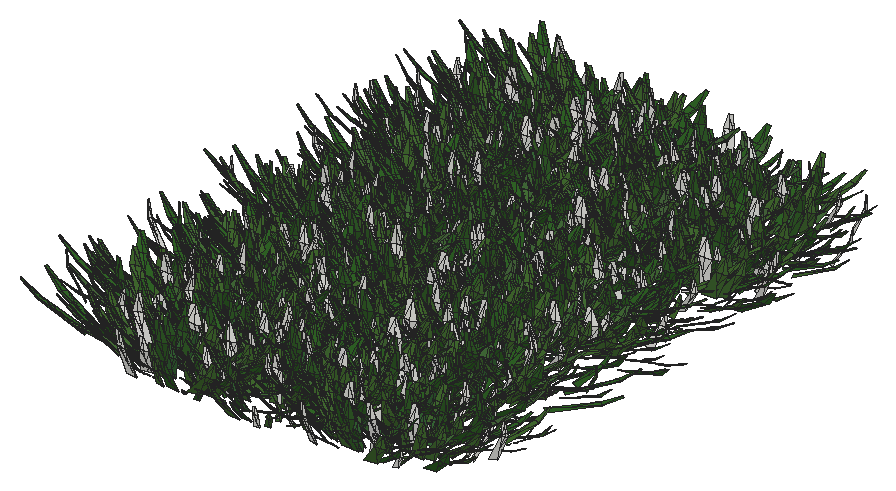
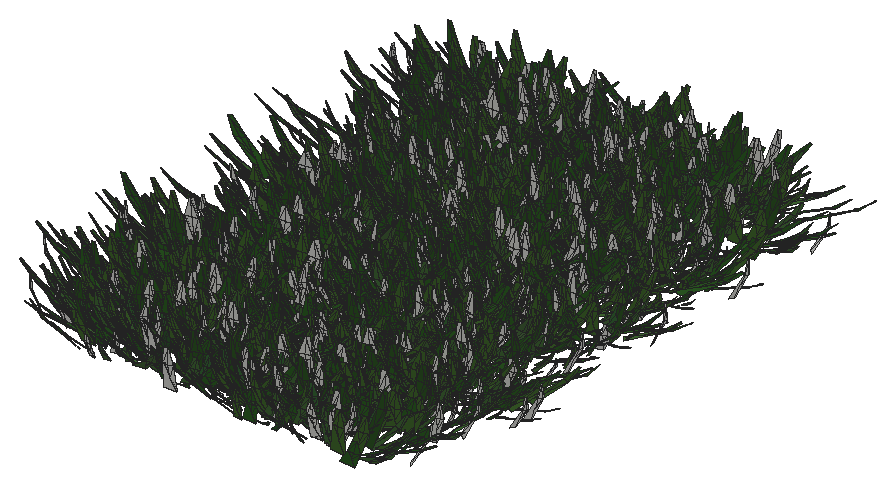
# SketchUp Ruby script. Lengths in inches.
U = 1.inch
M = Sketchup.active_model
def pt(a) = Geom::Point3d.new(a.map { |v| v * U })
def face(e, loops, mat)
  f = e.add_face(loops[0].map { |a| pt(a) })
  loops[1..].each { |l| e.add_face(l.map { |a| pt(a) }).erase! }
  f.material = f.back_material = mat if mat
  f
end
# faces: each face lists its corners as indices into pts; further lists are holes
def faces(e, pts, list, mat = nil) = list.each { |f| face(e, (f[0].is_a?(Array) ? f : [f]).map { |l| l.map { |i| pts[i] } }, mat) }
# xy, xz, yz: faces in a plane at the given z, y or x. An outline is a flat list of corners, or four numbers for a rectangle; further outlines are holes
def ring(l) = l.size == 4 ? [[l[0], l[1]], [l[2], l[1]], [l[2], l[3]], [l[0], l[3]]] : l.each_slice(2).to_a
def flat(e, list, mat, &to3) = list.each { |f| face(e, (f[0].is_a?(Array) ? f : [f]).map { |l| ring(l).map { |u, v| to3.(u, v) } }, mat) }
def xy(e, z, list, mat = nil) = flat(e, list, mat) { |x, y| [x, y, z] }
def xz(e, y, list, mat = nil) = flat(e, list, mat) { |x, z| [x, y, z] }
def yz(e, x, list, mat = nil) = flat(e, list, mat) { |y, z| [x, y, z] }
def lines(e, pts, list) = list.each { |a, b| e.add_line(pt(pts[a]), pt(pts[b])) }
# prism: a flat outline (further loops are holes) pulled along v
def prism(e, loops, v, mat = nil)
  f = face(e, loops, mat); d = Geom::Vector3d.new(v.map { |x| x * U })
  f.pushpull(f.normal.samedirection?(d) ? d.length : -d.length)
end
def box(e, o, s, mat = nil) = prism(e, [[o, [o[0] + s[0], o[1], o[2]], [o[0] + s[0], o[1] + s[1], o[2]], [o[0], o[1] + s[1], o[2]]]], [0, 0, s[2]], mat)
def at(x, y, z, deg = 0) = Geom::Transformation.translation(pt([x, y, z])) * Geom::Transformation.rotation(ORIGIN, Z_AXIS, deg.degrees)
def axes(o, x, y, z) = Geom::Transformation.new([*x, 0, *y, 0, *z, 0, *pt(o).to_a, 1])
def part(name) = M.definitions.add(name)
# library, detail: a bought-in or finely detailed component or shape, given as its bounding box
def library(name, o, s) = part(name).tap { |d| box(d.entities, o, s) }
def detail(e, o, s) = box(e.add_group.entities, o, s)
def put(e, d, t, mat = nil) = e.add_instance(d, t).tap { |i| i.material = mat if mat }
def group(e, t, mat = nil) = e.add_group.tap { |g| g.transformation = t; g.material = mat if mat }.entities
root = M.entities
M.materials.add("Material82").color = [68, 110, 58]
M.materials.add("Material83").color = [48, 90, 38]
M.materials.add("Material84").color = [68, 110, 48]
M.materials.add("Material85").color = [48, 90, 48]
M.materials.add("Material86").color = [58, 110, 58]
M.materials.add("Material87").color = [58, 90, 38]
M.materials.add("Material88").color = [68, 100, 58]
M.materials.add("Material89").color = [48, 100, 38]
c1 = part("grass00")
p = [[-0.6875,0.15,0],[-0.56,0.08,5.52],[-0.04,0.03,2.76],[0.48,-0.02,0],[0.35,-0.02,5.52],[-0.1,-0.14,5.52],
  [-0.12,0.65,8.37],[-0.42,0.65,8.37]]
faces(c1.entities,p,[[0,1,2,3],[3,2,4],[1,5,2],[5,4,2],[1,6,5],[4,5,6],[7,6,1]])
c2 = part("Group16\#1")
put(c2.entities,c1,axes([1.44,-0.61,-0.01],[0.05352,0.12609,0],[-0.10704,0.04543,0.07239],[0.06664,-0.02828,0.11628]),"Material85")
put(c2.entities,c1,axes([0.76,-0.15,-0.01],[0.04676,0.24062,0],[-0.23162,0.04501,0.06642],[0.0652,-0.01267,0.23595]),"Material82")
put(c2.entities,c1,axes([0.79,0.01,-0.01],[-0.00606,0.34651,0],[-0.34381,-0.00602,0.0432],[0.04319,0.00076,0.34386]))
put(c2.entities,c1,axes([1,0.23,-0.01],[-0.07192,0.31144,0],[-0.28722,-0.06632,0.1236],[0.12043,0.02781,0.29478]),"Material84")
put(c2.entities,c1,axes([1.66,0.77,-0.01],[-0.13828,0.29651,0],[-0.21551,-0.1005,0.22471],[0.20365,0.09498,0.23779]),"Material89")
put(c2.entities,c1,axes([0.6875,0.52,-0.01],[-0.18126,0.24051,0],[-0.22746,-0.17142,0.09788],[0.07817,0.05891,0.28481]),"Material84")
put(c2.entities,c1,axes([0.68,0.78,-0.01],[-0.215,0.18688,0],[-0.12385,-0.14248,0.21334],[0.13995,0.16101,0.18878]),"Material82")
put(c2.entities,c1,axes([0.56,1,-0.01],[-0.13756,0.07624,0],[-0.06159,-0.11112,0.0927],[0.04494,0.08108,0.12705]),"Material84")
put(c2.entities,c1,axes([0.2,0.64,-0.01],[-0.23729,0.07254,0],[-0.05711,-0.18681,0.153],[0.04473,0.14632,0.19535]),"Material89")
put(c2.entities,c1,axes([0.0625,0.72,-0.01],[-0.28874,0.02525,0],[-0.02179,-0.24916,0.14647],[0.01276,0.14591,0.25012]),"Material82")
put(c2.entities,c1,axes([-0.08,0.62,-0.01],[-0.34089,-0.04187,0],[0.03255,-0.26504,0.216],[-0.02633,0.21439,0.26703]),"Material89")
put(c2.entities,c1,axes([-0.34,0.98,-0.01],[-0.14314,-0.0493,0],[0.04397,-0.12769,0.06843],[-0.02228,0.0647,0.13505]),"Material89")
put(c2.entities,c1,axes([-0.87,1.45,-0.01],[-0.23488,-0.14114,0],[0.13761,-0.22901,0.06087],[-0.03135,0.05217,0.26717]))
put(c2.entities,c1,axes([-0.72,0.77,-0.01],[-0.14208,-0.13251,0],[0.07209,-0.0773,0.16301],[-0.11118,0.11922,0.1057]),"Material89")
put(c2.entities,c1,axes([-0.62,0.43,-0.01],[-0.14845,-0.21203,0],[0.18654,-0.13061,0.12304],[-0.10079,0.07057,0.22772]),"Material82")
put(c2.entities,c1,axes([-0.68,0.29,-0.01],[-0.13639,-0.32136,0],[0.31723,-0.13464,0.05579],[-0.05136,0.0218,0.34462]),"Material83")
put(c2.entities,c1,axes([-0.64,0.125,-0.01],[-0.0458,-0.23569,0],[0.22124,-0.043,0.08276],[-0.08124,0.01579,0.22538]),"Material86")
put(c2.entities,c1,axes([-1.6,-0.03,-0.01],[0.00576,-0.32897,0],[0.27526,0.00482,0.18018],[-0.18015,-0.00315,0.2753]),"Material84")
put(c2.entities,c1,axes([-1.36,-0.31,-0.01],[0.05718,-0.24765,0],[0.18172,0.04196,0.17267],[-0.16825,-0.03885,0.1865]),"Material89")
put(c2.entities,c1,axes([-1.54,-0.72,-0.01],[0.06537,-0.14017,0],[0.13555,0.06321,0.03939],[-0.0357,-0.01665,0.14956]))
put(c2.entities,c1,axes([-1.19,-0.9,-0.01],[0.09597,-0.12735,0],[0.11214,0.08451,0.07557],[-0.06035,-0.04548,0.14042]),"Material88")
put(c2.entities,c1,axes([-0.47,-0.54,-0.01],[0.11588,-0.10072,0],[0.0618,0.0711,0.12124],[-0.07953,-0.0915,0.0942]))
put(c2.entities,c1,axes([-0.47,-0.84,-0.01],[0.11927,-0.0661,0],[0.06603,0.11913,0.00646],[-0.00313,-0.00565,0.13621]),"Material84")
put(c2.entities,c1,axes([-0.38,-1.24,-0.01],[0.28037,-0.08571,0],[0.0618,0.20215,0.20315],[-0.05939,-0.19428,0.21139]),"Material88")
put(c2.entities,c1,axes([-0.06,-0.66,-0.01],[0.22719,-0.01987,0],[0.01247,0.14255,0.17758],[-0.01547,-0.17691,0.1431]),"Material87")
put(c2.entities,c1,axes([0.11,-0.89,-0.01],[0.14882,0.01828,0],[-0.01058,0.08611,0.12229],[0.01491,-0.12138,0.08676]),"Material85")
put(c2.entities,c1,axes([0.25,-0.72,-0.01],[0.20481,0.07053,0],[-0.06206,0.18022,0.10291],[0.03351,-0.0973,0.1906]),"Material85")
put(c2.entities,c1,axes([0.85,-1.42,-0.01],[0.16481,0.09904,0],[-0.09472,0.15762,0.05616],[0.02893,-0.04814,0.18389]),"Material84")
put(c2.entities,c1,axes([1.01,-1.09,-0.01],[0.21858,0.20385,0],[-0.17495,0.1876,0.15339],[0.10462,-0.11218,0.25652]),"Material89")
put(c2.entities,c1,axes([1.01,-0.71,-0.01],[0.08733,0.12473,0],[-0.06445,0.04512,0.13037],[0.1068,-0.07477,0.07867]),"Material85")
c3 = part("Group15\#1")
put(c3.entities,c2,at(0,0,0))
c4 = part("3darcstudiotree_grass00\#1")
put(c4.entities,c3,at(0,0,0))
put(root,c4,axes([746.18,955.9,-29.74],[2.02269,1.40625,0],[-2.88305,0.64496,-0.03898],[-0.27125,0.06068,1.98748]))
put(root,c4,axes([746.54,983.84,-29.74],[2.29641,1.07421,0],[-2.57105,0.85483,-0.04117],[-0.19383,0.06444,1.55213]))
put(root,c4,axes([746.51,946.6,-29.74],[0.20899,1.64265,0],[-4.27343,0.08456,-0.03261],[-0.1888,0.00374,1.85888]))
put(root,c4,axes([746.37,966.71,-29.74],[1.08869,1.44245,0],[-3.40274,0.39943,-0.00785],[-0.05372,0.00631,1.89978]))
put(root,c4,axes([746.58,981.94,-29.74],[2.7006,1.1614,0],[-2.43909,0.8821,-0.03804],[-0.19893,0.07194,1.7602]))
put(root,c4,axes([749.25,973.19,-29.74],[-2.45174,-1.03973,0],[2.50397,-0.91832,-0.03633],[0.18002,-0.06602,1.73438]))
put(root,c4,axes([749.35,970.78,-29.74],[-1.7758,-1.16797,0],[3.11451,-0.73649,-0.04451],[0.21848,-0.05166,1.55797]))
put(root,c4,axes([749.84,960.11,-29.74],[-4.0045,-0.70324,0],[1.53901,-1.36302,-0.04343],[0.08424,-0.0746,1.35201]))
put(root,c4,axes([749.58,953.62,-29.74],[-0.8562,-1.46222,0],[3.2715,-0.29793,-0.0292],[0.1741,-0.01586,1.53984]))
put(root,c4,axes([749.32,961.45,-29.74],[2.12424,-1.58648,0],[2.98317,0.62124,-0.03491],[0.20173,0.04201,1.65255]))
put(root,c4,axes([750.05,942.04,-29.74],[-3.45178,0.2701,0],[-0.90786,-1.80446,-0.05548],[-0.0508,-0.10098,1.6451]))
put(root,c4,axes([751.18,982.04,-29.74],[-3.12186,-1.16816,0],[2.84193,-1.18123,-0.00166],[0.00643,-0.00267,1.74215]))
put(root,c4,axes([749.34,988.83,-29.74],[3.25093,0.54248,0],[-1.41803,1.32165,-0.02719],[-0.07494,0.06985,1.929]))
put(root,c4,axes([749.35,989.51,-29.74],[-0.25702,1.50589,0],[-4.4334,-0.11768,-0.01753],[-0.09867,-0.00262,1.87889]))
put(root,c4,axes([749.26,967.875,-29.74],[3.97101,0.68213,0],[-1.55734,1.41002,-0.04191],[-0.07595,0.06876,1.32656]))
put(root,c4,axes([749.84,995.21,-29.74],[0.4621,1.41992,0],[-4.03416,0.20419,-0.0516],[-0.33532,0.01697,1.99718]))
put(root,c4,axes([749.66,977.52,-29.74],[4.12561,0.29265,0],[-0.72369,1.58676,-0.03729],[-0.0346,0.07587,1.60628]))
put(root,c4,axes([751.41,950.6,-29.74],[-3.96689,-0.26306,0],[0.64548,-1.51387,-0.0114],[0.01279,-0.03,1.97478]))
put(root,c4,axes([749.91,974.62,-29.74],[2.01819,1.66422,0],[-3.45385,0.65143,-0.02212],[-0.1358,0.02561,1.95299]))
put(root,c4,axes([750.19,958.22,-29.74],[-0.26486,1.49696,0],[-3.89065,-0.10706,-0.02357],[-0.1242,-0.00342,1.54387]))
put(root,c4,axes([750.2,948.51,-29.74],[4.24203,-0.02956,0],[0.08072,1.80172,-0.02875],[0.00231,0.05162,1.55972]))
put(root,c4,axes([750.35,983.97,-29.74],[2.46344,0.86677,0],[-2.31784,1.02455,-0.00625],[-0.02756,0.01218,1.72796]))
put(root,c4,axes([751.8,965.53,-29.74],[-3.7951,0.9119,0],[-2.12877,-1.37789,-0.05764],[-0.17628,-0.1141,1.8024]))
put(root,c4,axes([752.19,944.45,-29.74],[1.13972,-1.41461,0],[4.50389,0.56436,-0.03698],[0.18209,0.02282,1.82987]))
put(root,c4,axes([752.75,954.77,-29.74],[-2.49551,-1.26471,0],[2.8619,-0.87828,-0.01663],[0.09126,-0.02801,1.89037]))
put(root,c4,axes([752.39,940.35,-29.74],[-2.98133,1.10226,0],[-2.6348,-1.10837,-0.04557],[-0.21161,-0.08902,1.96028]))
put(root,c4,axes([752,978.84,-29.74],[-2.13819,1.22316,0],[-3.167,-0.86103,-0.02321],[-0.1127,-0.03064,1.70026]))
put(root,c4,axes([752.66,947.39,-29.74],[-3.3677,0.38425,0],[-1.22656,-1.67195,-0.00573],[-0.0077,-0.0105,1.59925]))
put(root,c4,axes([752.61,986.4,-29.74],[2.12809,-1.0558,0],[3.61722,1.13396,-0.06111],[0.24603,0.07713,1.78135]))
put(root,c4,axes([752.72,993.1,-29.74],[3.47556,-0.63984,0],[1.81232,1.53108,-0.02938],[0.06383,0.05392,1.64954]))
put(root,c4,axes([752.54,964.29,-29.74],[4.6709,-0.11713,0],[0.23839,1.47848,-0.03177],[0.01367,0.08477,1.90853]))
put(root,c4,axes([754.75,971.1,-29.74],[-3.65792,-0.8597,0],[1.995,-1.32021,-0.01663],[0.05672,-0.03754,1.94585]))
put(root,c4,axes([754.9,940.4,-29.74],[3.22982,-1.36398,0],[2.52221,0.92889,-0.01281],[0.05669,0.02088,1.56626]))
put(root,c4,axes([756.37,966.21,-29.74],[-1.61628,-1.19973,0],[3.67441,-0.7699,-0.00698],[0.03732,-0.00782,1.8873]))
put(root,c4,axes([756.01,944.1875,-29.74],[1.53079,-1.5017,0],[4.19952,0.6658,-0.01772],[0.08663,0.01374,1.7874]))
put(root,c4,axes([756.53,953.47,-29.74],[-3.12873,-1.31633,0],[2.88309,-1.0658,-0.03051],[0.12402,-0.04585,1.65027]))
put(root,c4,axes([755.92,991.84,-29.74],[2.10607,-1.53284,0],[3.55653,0.76,-0.00988],[0.05409,0.01156,1.88737]))
put(root,c4,axes([754.89,959.43,-29.74],[4.72899,0.01401,0],[-0.03317,1.74196,-0.012],[-0.00046,0.02441,1.70791]))
put(root,c4,axes([755.64,942.24,-29.74],[3.14565,-0.76847,0],[1.85222,1.17921,-0.00486],[0.01386,0.00882,1.42853]))
put(root,c4,axes([755.02,961.83,-29.74],[1.47307,1.52241,0],[-3.55442,0.5349,-0.03212],[-0.18221,0.02742,1.73128]))
put(root,c4,axes([755.39,948.7,-29.74],[3.86384,0.07818,0],[-0.23972,1.84255,-0.05168],[-0.01275,0.09801,1.68853]))
put(root,c4,axes([755.23,955.48,-29.74],[0.17144,1.84869,0],[-4.60552,0.06643,-0.0182],[-0.07619,0.0011,1.44668]))
put(root,c4,axes([755.38,974.37,-29.74],[0.6087,1.43701,0],[-3.38203,0.22281,-0.00028],[-0.00164,0.00011,1.50491]))
put(root,c4,axes([755.7,990.32,-29.74],[-0.11554,1.45354,0],[-4.02615,-0.04978,-0.04067],[-0.20655,-0.00255,1.53414]))
put(root,c4,axes([756.52,981.89,-29.74],[-3.14808,1.22755,0],[-2.57668,-1.02773,-0.03762],[-0.14164,-0.05649,1.47105]))
put(root,c4,axes([755.37,986.65,-29.74],[0.48824,1.58889,0],[-4.56618,0.21822,-0.01569],[-0.06712,0.00321,1.48562]))
put(root,c4,axes([757.53,977.55,-29.74],[-3.3453,-1.30601,0],[3.28392,-1.30825,-0.03717],[0.14464,-0.05762,1.93537]))
put(root,c4,axes([757.32,972.4,-29.74],[-4.03093,-0.26709,0],[0.61626,-1.44652,-0.01654],[0.01865,-0.04378,1.89711]))
put(root,c4,axes([757.72,978.98,-29.74],[-1.63649,-1.29377,0],[3.38922,-0.66676,-0.00448],[0.02699,-0.00531,1.90991]))
put(root,c4,axes([756.9,958.33,-29.74],[-3.19374,0.7238,0],[-2.32014,-1.59223,-0.04948],[-0.1132,-0.07768,1.60238]))
put(root,c4,axes([756.35,984.03,-29.74],[0.67214,1.30105,0],[-3.68417,0.29602,-0.04728],[-0.27019,0.02171,1.64346]))
put(root,c4,axes([756.68,968.28,-29.74],[3.23921,0.6316,0],[-1.61427,1.28761,-0.03066],[-0.08714,0.06951,1.75054]))
put(root,c4,axes([757.78,947.34,-29.74],[0.38628,-1.42854,0],[3.50239,0.14729,-0.04937],[0.32013,0.01346,1.72169]))
put(root,c4,axes([758.01,963.77,-29.74],[-1.61807,1.52118,0],[-3.6405,-0.60227,-0.04701],[-0.26943,-0.04457,1.83905]))
put(root,c4,axes([758.2,951.08,-29.74],[0.41177,1.61489,0],[-3.5087,0.13914,-0.04963],[-0.27633,0.01096,1.47912]))
put(root,c4,axes([757.57,994.14,-29.74],[3.03872,1.12896,0],[-3.11924,1.30579,-0.01047],[-0.04051,0.01696,1.92288]))
put(root,c4,axes([758.61,987.59,-29.74],[3.86781,0.52244,0],[-1.13731,1.30954,-0.02009],[-0.0432,0.04974,1.7458]))
put(root,c4,axes([760.32,986.48,-29.74],[-4.0386,-0.4374,0],[0.94795,-1.36128,-0.02848],[0.0516,-0.0741,1.83531]))
put(root,c4,axes([760.06,992.54,-29.74],[-0.39879,-1.78911,0],[3.98788,-0.13825,-0.04765],[0.27848,-0.00965,1.76037]))
put(root,c4,axes([760.28,995.03,-29.74],[-3.75498,0.92244,0],[-1.75834,-1.11323,-0.01072],[-0.04199,-0.02659,1.84718]))
put(root,c4,axes([760.82,955.28,-29.74],[-3.9685,0.8355,0],[-2.02289,-1.49439,-0.03463],[-0.09424,-0.06962,1.86049]))
put(root,c4,axes([760.41,962.1875,-29.74],[-1.70053,1.52985,0],[-3.13018,-0.54115,-0.01229],[-0.08699,-0.01504,1.9803]))
put(root,c4,axes([761.82,983.63,-29.74],[-3.28059,-1.08182,0],[2.91353,-1.37413,-0.04137],[0.10673,-0.05034,1.36909]))
put(root,c4,axes([761.33,975.17,-29.74],[3.17929,-0.7211,0],[2.23361,1.53163,-0.03788],[0.07878,0.05402,1.40078]))
put(root,c4,axes([760.76,972.49,-29.74],[4.05026,0.33604,0],[-0.7921,1.48485,-0.04482],[-0.0484,0.09073,1.51278]))
put(root,c4,axes([762.53,987.75,-29.74],[-2.84597,-0.98358,0],[2.28129,-1.02662,-0.01406],[0.06335,-0.02851,1.77353]))
put(root,c4,axes([761.69,981.77,-29.74],[3.81863,-0.53813,0],[1.40932,1.55539,-0.0155],[0.0332,0.03664,1.9985]))
put(root,c4,axes([763.01,949.61,-29.74],[-2.42754,-1.16571,0],[2.71881,-0.88058,-0.021],[0.08634,-0.02796,1.40308]))
put(root,c4,axes([762.95,956.96,-29.74],[-1.73285,-1.40976,0],[3.20349,-0.61242,-0.03263],[0.20579,-0.03934,1.87]))
put(root,c4,axes([761.86,979.68,-29.74],[3.58142,-0.447,0],[1.06233,1.32378,-0.04021],[0.07095,0.08841,1.5432]))
put(root,c4,axes([763.12,953.95,-29.74],[-4.30499,0.20084,0],[-0.50439,-1.68151,-0.02284],[-0.01208,-0.04026,1.44864]))
put(root,c4,axes([762.57,946.27,-29.74],[-2.18902,1.07825,0],[-2.9207,-0.92221,-0.02462],[-0.13408,-0.04234,1.95656]))
put(root,c4,axes([762,942.99,-29.74],[2.94971,1.39882,0],[-3.26889,1.07209,-0.02991],[-0.14108,0.04627,1.95467]))
put(root,c4,axes([763.86,964.38,-29.74],[0.02605,-1.38879,0],[4.64619,0.01356,-0.04606],[0.23946,0.0007,1.81052]))
put(root,c4,axes([762.28,966.1,-29.74],[3.34775,0.73741,0],[-1.81639,1.28251,-0.02091],[-0.0568,0.0401,1.55496]))
put(root,c4,axes([762.1875,977.25,-29.74],[4.2068,0.84458,0],[-2.08885,1.6182,-0.01612],[-0.03432,0.02659,1.61949]))
put(root,c4,axes([763.64,969.12,-29.74],[-3.54698,0.73807,0],[-1.81276,-1.35492,-0.01893],[-0.04162,-0.0311,1.37131]))
put(root,c4,axes([763.66,944.96,-29.74],[-3.36311,0.85521,0],[-1.93534,-1.1837,-0.01497],[-0.0443,-0.0271,1.4615]))
put(root,c4,axes([763.03,940.16,-29.74],[0.45304,1.69594,0],[-3.37186,0.14009,-0.01763],[-0.11097,0.00461,1.60818]))
put(root,c4,axes([763.26,970.46,-29.74],[2.84839,1.04367,0],[-2.27167,0.96426,-0.03885],[-0.20657,0.08768,1.95422]))
put(root,c4,axes([763.78,989.98,-29.74],[3.6343,-0.40762,0],[1.19135,1.65202,-0.03545],[0.05267,0.07304,1.77295]))
put(root,c4,axes([763.49,959.63,-29.74],[0.87217,1.79185,0],[-4.36686,0.33058,-0.02457],[-0.1156,0.00875,1.59681]))
put(root,c4,axes([764.07,950.48,-29.74],[3.8213,1.10557,0],[-2.37941,1.27911,-0.00415],[-0.01079,0.0058,1.32509]))
put(root,c4,axes([765.6,955.88,-29.74],[1.36885,-1.43158,0],[3.98655,0.59286,-0.04892],[0.27754,0.04127,1.93615]))
put(root,c4,axes([766.26,975.04,-29.74],[-3.05635,-0.6343,0],[1.70161,-1.2752,-0.01604],[0.05188,-0.03888,1.9024]))
put(root,c4,axes([766.42,983.79,-29.74],[-0.79946,-1.53657,0],[4.27905,-0.34626,-0.03341],[0.18605,-0.01506,1.86102]))
put(root,c4,axes([766.06,953.25,-29.74],[1.53865,-1.45346,0],[4.25105,0.69992,-0.03949],[0.18935,0.03118,1.7941]))
put(root,c4,axes([766.71,967.02,-29.74],[-2.53143,-1.15701,0],[3.22557,-1.09761,-0.03179],[0.10043,-0.03417,1.33245]))
put(root,c4,axes([767.22,978.59,-29.74],[0.41929,-1.46273,0],[4.6699,0.2082,-0.01256],[0.06761,0.00301,1.90836]))
put(root,c4,axes([765.6875,945.1,-29.74],[3.57437,0.42668,0],[-1.04232,1.35805,-0.0422],[-0.08519,0.111,1.87907]))
put(root,c4,axes([766.11,967.68,-29.74],[4.54472,-0.07638,0],[0.17813,1.64846,-0.04096],[0.00957,0.08859,1.72127]))
put(root,c4,axes([767.89,959.96,-29.74],[-1.16799,-1.2811,0],[3.57696,-0.50721,-0.0171],[0.1013,-0.01436,1.79343]))
put(root,c4,axes([767.52,992.61,-29.74],[-4.37429,0.70017,0],[-1.56113,-1.51689,-0.01879],[-0.03338,-0.03243,1.46955]))
put(root,c4,axes([767.85,951.32,-29.74],[-3.24054,-0.28468,0],[0.77392,-1.37016,-0.02543],[0.03342,-0.05916,1.61262]))
put(root,c4,axes([767.28,981.88,-29.74],[-2.88569,0.96312,0],[-2.81786,-1.31311,-0.05904],[-0.17262,-0.08044,1.47981]))
put(root,c4,axes([768.06,948.71,-29.74],[1.16933,-1.48396,0],[3.883,0.47588,-0.02169],[0.1048,0.01284,1.54236]))
put(root,c4,axes([768.51,945.8125,-29.74],[-0.65586,-1.46962,0],[4.60144,-0.31938,-0.05842],[0.32577,-0.02261,1.98292]))
put(root,c4,axes([767.71,971.44,-29.74],[3.94842,-0.68884,0],[1.45256,1.29494,-0.00969],[0.01982,0.01767,1.36001]))
put(root,c4,axes([769.05,963.67,-29.74],[-3.73914,-0.79189,0],[1.71097,-1.25649,-0.0264],[0.09118,-0.06696,1.979]))
put(root,c4,axes([768.89,989.64,-29.74],[-3.92506,-0.07313,0],[0.21494,-1.79423,-0.03065],[0.00834,-0.06965,1.9691]))
put(root,c4,axes([767.29,973.37,-29.74],[4.38423,0.4309,0],[-1.14012,1.80418,-0.03274],[-0.03634,0.0575,1.62193]))
put(root,c4,axes([769.19,957.5,-29.74],[-3.57377,-0.68668,0],[1.88387,-1.52489,-0.02869],[0.074,-0.0599,1.89824]))
put(root,c4,axes([767.69,961.16,-29.74],[4.39904,-0.03006,0],[0.06093,1.38656,-0.04649],[0.00481,0.10943,1.57333]))
put(root,c4,axes([768.45,994.33,-29.74],[3.99314,-0.58395,0],[1.40862,1.49812,-0.01564],[0.03379,0.03593,1.88746]))
put(root,c4,axes([768.56,987.28,-29.74],[-1.29956,1.24249,0],[-3.63161,-0.59077,-0.01866],[-0.09119,-0.01483,1.55626]))
put(root,c4,axes([769.16,976.875,-29.74],[4.62104,-0.01455,0],[0.03483,1.71996,-0.00522],[0.00018,0.00901,1.42947]))
put(root,c4,axes([769.35,985.5,-29.74],[1.74244,1.18271,0],[-3.27168,0.74965,-0.03711],[-0.19162,0.04391,1.69359]))
put(root,c4,axes([769.2,941.69,-29.74],[2.60331,1.05125,0],[-2.58261,0.9947,-0.01838],[-0.08057,0.03103,1.65818]))
put(root,c4,axes([771.32,962.15,-29.74],[-4.17671,-0.8199,0],[2.05439,-1.62767,-0.0574],[0.10467,-0.08292,1.41402]))
put(root,c4,axes([771.65,992.11,-29.74],[-3.98486,0.06108,0],[-0.1339,-1.35868,-0.04521],[-0.01298,-0.1317,1.91035]))
put(root,c4,axes([772.08,981.68,-29.74],[-3.51388,-0.90483,0],[2.14031,-1.29273,-0.0556],[0.17294,-0.10445,1.66946]))
put(root,c4,axes([771.14,968.93,-29.74],[-2.56609,1.18757,0],[-3.37526,-1.13431,-0.01912],[-0.05922,-0.0199,1.35238]))
put(root,c4,axes([772.33,950.59,-29.74],[-3.1974,-0.52057,0],[1.31873,-1.25975,-0.01181],[0.03016,-0.02882,1.73426]))
put(root,c4,axes([772.18,959.85,-29.74],[-0.51556,-1.46046,0],[3.95081,-0.21691,-0.04493],[0.28513,-0.01565,1.91565]))
put(root,c4,axes([772.26,989.8125,-29.74],[0.81424,-1.34129,0],[3.64589,0.34423,-0.00366],[0.01919,0.00181,1.51551]))
put(root,c4,axes([772.79,949.61,-29.74],[0.21445,-1.64927,0],[3.6182,0.07317,-0.01161],[0.06174,0.00125,1.44612]))
put(root,c4,axes([773.41,975.71,-29.74],[-3.21256,-1.12789,0],[2.70503,-1.19832,-0.03256],[0.11538,-0.05111,1.62483]))
put(root,c4,axes([773.5,979.87,-29.74],[-3.59955,0.15303,0],[-0.4164,-1.52331,-0.01956],[-0.01422,-0.05201,1.97453]))
put(root,c4,axes([772.24,942.38,-29.74],[-0.10583,1.54224,0],[-3.7996,-0.04055,-0.00627],[-0.03571,-0.00038,1.62459]))
put(root,c4,axes([774.01,994.14,-29.74],[-2.41013,-1.27132,0],[2.91819,-0.86042,-0.02089],[0.0972,-0.02866,1.58683]))
put(root,c4,axes([773.39,955.47,-29.74],[-3.10318,1.24143,0],[-2.60712,-1.01358,-0.05097],[-0.2393,-0.09303,1.80901]))
put(root,c4,axes([773.01,940.45,-29.74],[-1.86859,1.14232,0],[-3.14905,-0.80116,-0.00439],[-0.02189,-0.00557,1.66469]))
put(root,c4,axes([772.99,988.09,-29.74],[-1.19351,1.65501,0],[-3.6228,-0.40633,-0.01558],[-0.10093,-0.01132,1.90128]))
put(root,c4,axes([772.59,965.58,-29.74],[3.31436,0.96989,0],[-2.30719,1.22623,-0.02502],[-0.09786,0.05201,1.90511]))
put(root,c4,axes([774.63,985.85,-29.74],[-1.03972,-1.40109,0],[4.3795,-0.50546,-0.04795],[0.2061,-0.02379,1.53186]))
put(root,c4,axes([773.18,946.2,-29.74],[-0.80891,1.58211,0],[-4.50454,-0.3582,-0.03197],[-0.1625,-0.01292,1.78572]))
put(root,c4,axes([774.49,944.49,-29.74],[-3.61232,0.8121,0],[-2.24589,-1.55373,-0.01918],[-0.05035,-0.03483,1.80194]))
put(root,c4,axes([774.54,963.6,-29.74],[1.76506,-1.25364,0],[3.37171,0.73833,-0.03203],[0.17156,0.03757,1.771]))
put(root,c4,axes([774.43,984.46,-29.74],[-2.8527,1.28628,0],[-3.36111,-1.15935,-0.03347],[-0.14409,-0.0497,1.91416]))
put(root,c4,axes([773.87,956.76,-29.74],[4.4529,0.04613,0],[-0.09862,1.48061,-0.04419],[-0.00818,0.12282,1.98467]))
put(root,c4,axes([775.22,977.03,-29.74],[-4.01452,0.69277,0],[-1.67449,-1.50916,-0.02625],[-0.04914,-0.04429,1.46233]))
put(root,c4,axes([774.43,970.14,-29.74],[-0.38971,1.40175,0],[-3.70548,-0.16023,-0.02456],[-0.14917,-0.00645,1.70727]))
put(root,c4,axes([774.38,953.01,-29.74],[4.64374,0.18316,0],[-0.43015,1.69615,-0.02551],[-0.01161,0.04577,1.48132]))
put(root,c4,axes([774.96,972.26,-29.74],[3.33641,-0.4539,0],[1.10224,1.26009,-0.03311],[0.06709,0.0767,1.57439]))
put(root,c4,axes([777.125,984.49,-29.74],[-4.08837,-0.48406,0],[1.24556,-1.63618,-0.01736],[0.02056,-0.027,1.33702]))
put(root,c4,axes([776.95,965.96,-29.74],[1.677,-1.55355,0],[4.28787,0.71988,-0.03539],[0.14144,0.02375,1.51703]))
put(root,c4,axes([777.4,981.15,-29.74],[-2.71685,-1.17622,0],[2.71806,-0.97644,-0.02128],[0.11147,-0.04005,1.95268]))
put(root,c4,axes([777.65,945.82,-29.74],[-3.01218,-1.1682,0],[2.32929,-0.93411,-0.00764],[0.03903,-0.01565,1.81511]))
put(root,c4,axes([777.6875,992.61,-29.74],[0.25601,-1.60576,0],[3.7655,0.09337,-0.00515],[0.03185,0.00079,1.75106]))
put(root,c4,axes([776.7,971.13,-29.74],[-1.88352,1.24088,0],[-3.53635,-0.83485,-0.03562],[-0.13641,-0.0322,1.37892]))
put(root,c4,axes([777.42,943.02,-29.74],[0.35251,-1.39793,0],[3.51175,0.13773,-0.03727],[0.24286,0.00952,1.73202]))
put(root,c4,axes([777.6875,948.76,-29.74],[-3.43821,0.20499,0],[-0.69374,-1.80975,-0.03474],[-0.02131,-0.0556,1.42794]))
put(root,c4,axes([776.75,957.77,-29.74],[-0.07716,1.61232,0],[-4.08051,-0.03037,-0.05443],[-0.27918,-0.00208,1.56933]))
put(root,c4,axes([778.29,979.31,-29.74],[1.28288,-1.22527,0],[4.05082,0.65965,-0.04448],[0.2416,0.03934,1.93016]))
put(root,c4,axes([778.5625,987.7,-29.74],[-0.2981,-1.54731,0],[4.18924,-0.12553,-0.05563],[0.33136,-0.00993,1.88098]))
